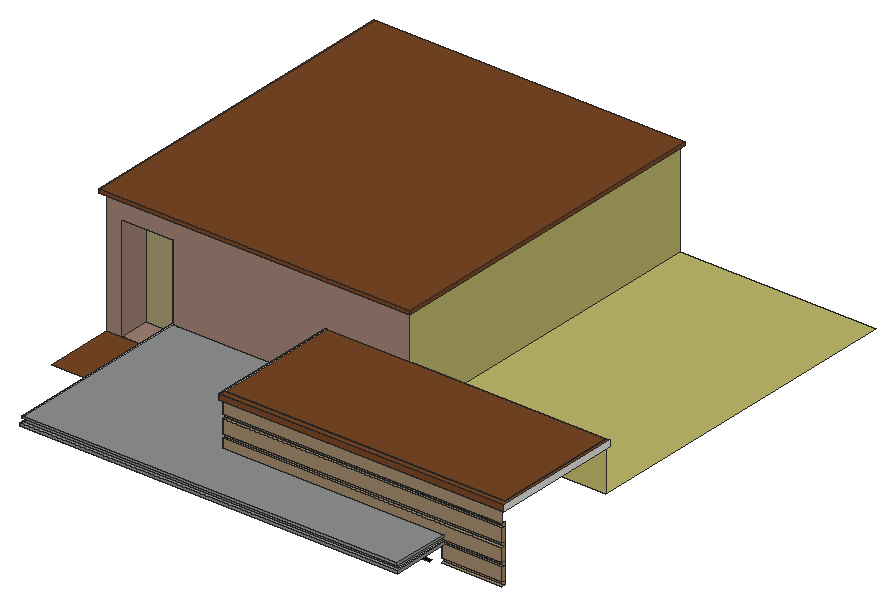
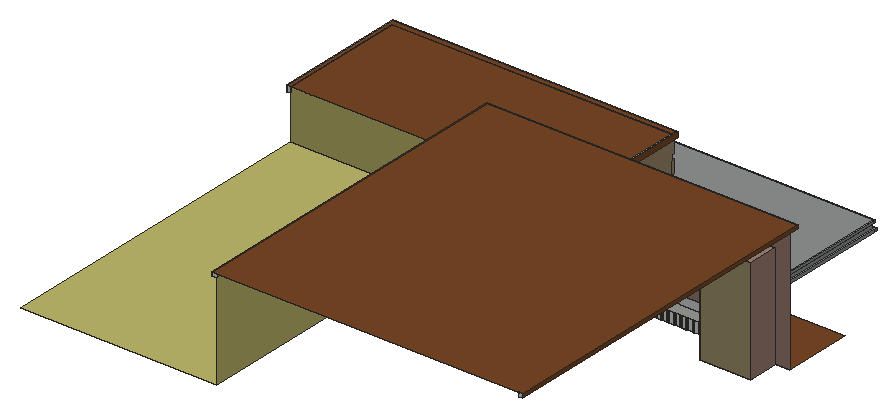
# SketchUp Ruby script. Lengths in inches.
U = 1.inch
M = Sketchup.active_model
def pt(a) = Geom::Point3d.new(a.map { |v| v * U })
def face(e, loops, mat)
  f = e.add_face(loops[0].map { |a| pt(a) })
  loops[1..].each { |l| e.add_face(l.map { |a| pt(a) }).erase! }
  f.material = f.back_material = mat if mat
  f
end
# faces: each face lists its corners as indices into pts; further lists are holes
def faces(e, pts, list, mat = nil) = list.each { |f| face(e, (f[0].is_a?(Array) ? f : [f]).map { |l| l.map { |i| pts[i] } }, mat) }
# xy, xz, yz: faces in a plane at the given z, y or x. An outline is a flat list of corners, or four numbers for a rectangle; further outlines are holes
def ring(l) = l.size == 4 ? [[l[0], l[1]], [l[2], l[1]], [l[2], l[3]], [l[0], l[3]]] : l.each_slice(2).to_a
def flat(e, list, mat, &to3) = list.each { |f| face(e, (f[0].is_a?(Array) ? f : [f]).map { |l| ring(l).map { |u, v| to3.(u, v) } }, mat) }
def xy(e, z, list, mat = nil) = flat(e, list, mat) { |x, y| [x, y, z] }
def xz(e, y, list, mat = nil) = flat(e, list, mat) { |x, z| [x, y, z] }
def yz(e, x, list, mat = nil) = flat(e, list, mat) { |y, z| [x, y, z] }
def lines(e, pts, list) = list.each { |a, b| e.add_line(pt(pts[a]), pt(pts[b])) }
# prism: a flat outline (further loops are holes) pulled along v
def prism(e, loops, v, mat = nil)
  f = face(e, loops, mat); d = Geom::Vector3d.new(v.map { |x| x * U })
  f.pushpull(f.normal.samedirection?(d) ? d.length : -d.length)
end
def box(e, o, s, mat = nil) = prism(e, [[o, [o[0] + s[0], o[1], o[2]], [o[0] + s[0], o[1] + s[1], o[2]], [o[0], o[1] + s[1], o[2]]]], [0, 0, s[2]], mat)
def at(x, y, z, deg = 0) = Geom::Transformation.translation(pt([x, y, z])) * Geom::Transformation.rotation(ORIGIN, Z_AXIS, deg.degrees)
def axes(o, x, y, z) = Geom::Transformation.new([*x, 0, *y, 0, *z, 0, *pt(o).to_a, 1])
def part(name) = M.definitions.add(name)
# library, detail: a bought-in or finely detailed component or shape, given as its bounding box
def library(name, o, s) = part(name).tap { |d| box(d.entities, o, s) }
def detail(e, o, s) = box(e.add_group.entities, o, s)
def put(e, d, t, mat = nil) = e.add_instance(d, t).tap { |i| i.material = mat if mat }
def group(e, t, mat = nil) = e.add_group.tap { |g| g.transformation = t; g.material = mat if mat }.entities
root = M.entities
M.materials.add("Niraj_Hair_Dark").color = [109, 109, 109]
M.materials.add("Niraj_Skin").color = [158, 128, 115]
M.materials.add("[0026_LightSalmon]").color = [255, 160, 122]
M.materials.add("[0035_Tan]").color = [158, 135, 105]
M.materials.add("[0057_DarkKhaki]").color = [189, 183, 107]
M.materials.add("[0137_Black]").color = [0, 0, 0]
M.materials.add("[Blacktop Old 02]").color = [143, 145, 145]
M.materials.add("[Wood Lumber ButtJoined]").color = [164, 152, 112]
M.materials.add("[Wood Veneer 01]").color = [120, 70, 37]
xy(root,249,[[18.5,262.5,71.22,294.13]],"Niraj_Skin")
xy(root,249.09,[[71.42,259.5,75.97,262.5],[77.92,259.5,82.47,262.5],[84.42,259.5,88.97,262.5],[90.92,259.5,95.47,262.5],[97.42,259.5,101.97,262.5],
  [103.92,259.5,108.47,262.5],[110.42,259.5,114.97,262.5],[116.92,259.5,121.47,262.5],[123.42,259.5,127.97,262.5],[129.92,259.5,134.47,262.5],
  [136.42,259.5,140.97,262.5],[142.92,259.5,147.47,262.5],[149.42,259.5,153.97,262.5],[155.92,259.5,160.47,262.5],[162.42,259.5,166.97,262.5],
  [168.92,259.5,173.47,262.5],[175.17,259.5,179.72,262.5],[181.42,259.5,185.97,262.5],[187.67,259.5,192.22,262.5],[193.92,259.5,198.47,262.5],
  [200.17,259.5,204.72,262.5],[206.42,259.5,210.97,262.5],[212.67,259.5,217.22,262.5],[218.92,259.5,223.47,262.5],[225.17,259.5,229.72,262.5],
  [231.42,259.5,235.97,262.5],[237.67,259.5,242.22,262.5],[243.92,259.5,248.47,262.5],[250.17,259.5,254.72,262.5],[256.42,259.5,260.97,262.5],
  [262.67,259.5,267.22,262.5],[269.11,259.5,273.65,262.5],[275.54,259.5,280.09,262.5],[281.98,259.5,286.53,262.5],[288.42,259.5,292.97,262.5],
  [294.86,259.5,299.4,262.5],[301.29,259.5,305.84,262.5]])
xy(root,249.09,[[3.5,191.32,310.1875,191.32,310.1875,262.5,305.84,262.5,305.84,259.5,301.29,259.5,301.29,262.5,299.4,262.5,299.4,259.5,294.86,259.5,294.86,262.5,292.97,262.5,292.97,259.5,288.42,259.5,288.42,262.5,286.53,262.5,286.53,259.5,281.98,259.5,281.98,262.5,280.09,262.5,280.09,259.5,275.54,259.5,275.54,262.5,273.65,262.5,273.65,259.5,269.11,259.5,269.11,262.5,267.22,262.5,267.22,259.5,262.67,259.5,262.67,262.5,260.97,262.5,260.97,259.5,256.42,259.5,256.42,262.5,254.72,262.5,254.72,259.5,250.17,259.5,250.17,262.5,248.47,262.5,248.47,259.5,243.92,259.5,243.92,262.5,242.22,262.5,242.22,259.5,237.67,259.5,237.67,262.5,235.97,262.5,235.97,259.5,231.42,259.5,231.42,262.5,229.72,262.5,229.72,259.5,225.17,259.5,225.17,262.5,223.47,262.5,223.47,259.5,218.92,259.5,218.92,262.5,217.22,262.5,217.22,259.5,212.67,259.5,212.67,262.5,210.97,262.5,210.97,259.5,206.42,259.5,206.42,262.5,204.72,262.5,204.72,259.5,200.17,259.5,200.17,262.5,198.47,262.5,198.47,259.5,193.92,259.5,193.92,262.5,192.22,262.5,192.22,259.5,187.67,259.5,187.67,262.5,185.97,262.5,185.97,259.5,181.42,259.5,181.42,262.5,179.72,262.5,179.72,259.5,175.17,259.5,175.17,262.5,173.47,262.5,173.47,259.5,168.92,259.5,168.92,262.5,166.97,262.5,166.97,259.5,162.42,259.5,162.42,262.5,160.47,262.5,160.47,259.5,155.92,259.5,155.92,262.5,153.97,262.5,153.97,259.5,149.42,259.5,149.42,262.5,147.47,262.5,147.47,259.5,142.92,259.5,142.92,262.5,140.97,262.5,140.97,259.5,136.42,259.5,136.42,262.5,134.47,262.5,134.47,259.5,129.92,259.5,129.92,262.5,127.97,262.5,127.97,259.5,123.42,259.5,123.42,262.5,121.47,262.5,121.47,259.5,116.92,259.5,116.92,262.5,114.97,262.5,114.97,259.5,110.42,259.5,110.42,262.5,108.47,262.5,108.47,259.5,103.92,259.5,103.92,262.5,101.97,262.5,101.97,259.5,97.42,259.5,97.42,262.5,95.47,262.5,95.47,259.5,90.92,259.5,90.92,262.5,88.97,262.5,88.97,259.5,84.42,259.5,84.42,262.5,82.47,262.5,82.47,259.5,77.92,259.5,77.92,262.5,75.97,262.5,75.97,259.5,71.42,259.5,71.42,262.5,3.5,262.5]],"[Wood Veneer 01]")
xy(root,249.27,[[367.23,128.5,444.17,131.5]],"[0137_Black]")
xy(root,252.4375,[[456.23,128.5,518.75,131.5]],"[0035_Tan]")
xy(root,256.58,[[456.23,128.5,518.75,131.5]],"[0035_Tan]")
xy(root,269.38,[[71.42,259.5,75.97,262.5],[77.92,259.5,82.47,262.5],[84.42,259.5,88.97,262.5],[90.92,259.5,95.47,262.5],[97.42,259.5,101.97,262.5],
  [103.92,259.5,108.47,262.5],[110.42,259.5,114.97,262.5],[116.92,259.5,121.47,262.5],[123.42,259.5,127.97,262.5],[129.92,259.5,134.47,262.5],
  [136.42,259.5,140.97,262.5],[142.92,259.5,147.47,262.5],[149.42,259.5,153.97,262.5],[155.92,259.5,160.47,262.5],[162.42,259.5,166.97,262.5],
  [168.92,259.5,173.47,262.5],[175.17,259.5,179.72,262.5],[181.42,259.5,185.97,262.5],[187.67,259.5,192.22,262.5],[193.92,259.5,198.47,262.5],
  [200.17,259.5,204.72,262.5],[206.42,259.5,210.97,262.5],[212.67,259.5,217.22,262.5],[218.92,259.5,223.47,262.5],[225.17,259.5,229.72,262.5],
  [231.42,259.5,235.97,262.5],[237.67,259.5,242.22,262.5],[243.92,259.5,248.47,262.5],[250.17,259.5,254.72,262.5],[256.42,259.5,260.97,262.5],
  [262.67,259.5,267.22,262.5],[269.11,259.5,273.65,262.5],[275.54,259.5,280.09,262.5],[281.98,259.5,286.53,262.5],[288.42,259.5,292.97,262.5],
  [294.86,259.5,299.4,262.5],[301.29,259.5,305.84,262.5]])
xy(root,269.38,[[69.11,68.5,69.11,262.5,71.42,262.5,71.42,259.5,75.97,259.5,75.97,262.5,77.04,262.5,77.04,274.5,310.1875,274.5,310.1875,131.5,445.29,131.5,445.29,71.5,456.23,71.5,456.23,128.5,458.66,128.5,458.66,68.5]],"[Blacktop Old 02]")
xy(root,270.4375,[[456.23,128.5,518.75,131.5]],"[0035_Tan]")
xy(root,272.21,[[69.11,68.5,458.66,68.5,458.66,128.5,456.23,128.5,456.23,71.5,71.42,71.5,71.42,262.5,69.11,262.5]],"[Blacktop Old 02]")
xy(root,274.58,[[456.23,128.5,518.75,131.5]],"[0035_Tan]")
xy(root,276.6875,[[70.17,68.5,70.17,262.5,71.42,262.5,71.42,71.5,456.23,71.5,456.23,128.5,457.98,128.5,457.98,68.5]],"Niraj_Hair_Dark")
xy(root,279,[[230.1,128.5,456.23,131.5]])
xy(root,279,[[70.17,68.5,71.42,71.5]],"Niraj_Hair_Dark")
xy(root,279,[[316.1875,262.5,518.75,611.5]],"[0057_DarkKhaki]")
xy(root,279,[[71.42,68.5,457.98,68.5,457.98,128.5,230.1,128.5,230.1,262.5,310.1875,262.5,310.1875,274.5,77.04,274.5,77.04,262.5,71.42,262.5],[70.17,71.5,71.42,262.5]],"[Blacktop Old 02]")
xy(root,288.4375,[[230.1,128.5,518.75,131.5]],"[0035_Tan]")
xy(root,292.58,[[230.1,128.5,518.75,131.5]],"[0035_Tan]")
xy(root,306.4375,[[230.1,128.5,518.75,131.5]],"[0035_Tan]")
xy(root,310.58,[[230.1,128.5,518.75,131.5]],"[0035_Tan]")
xy(root,324.4375,[[230.1,128.5,518.75,131.5]])
xy(root,324.4375,[[228.35,125.5,228.35,262.5,230.1,262.5,230.1,128.5,518.75,128.5,518.75,262.5,522.9375,262.5,522.9375,125.5]],"[Wood Veneer 01]")
xy(root,330.3125,[[228.35,125.5,230.1,131.5],[230.1,125.5,522.9375,125.5,522.9375,262.5,518.75,262.5,518.75,131.5,230.1,131.5],[228.35,131.5,230.1,262.5],[230.1,131.5,518.75,262.5]],"[Wood Veneer 01]")
xy(root,357,[[18.5,262.5,71.22,294.13]],"Niraj_Skin")
xy(root,377.89,[[0,256.5,0,611.5,3.5,611.5,3.5,262.5,316.1875,262.5,316.1875,611.5,320.5,611.5,320.5,256.5]],"[Wood Veneer 01]")
xy(root,381.875,[[0,256.5,320.5,611.5]],"[Wood Veneer 01]")
xz(root,68.5,[[69.11,269.38,458.66,272.21],[70.17,276.6875,457.98,279]],"[Blacktop Old 02]")
xz(root,71.5,[[71.42,272.21,456.23,276.6875]],"[Blacktop Old 02]")
xz(root,125.5,[[228.35,324.4375,522.9375,330.3125]],"[Wood Veneer 01]")
xz(root,128.5,[[456.23,269.38,458.66,270.4375],[456.23,270.4375,458.66,272.21]])
xz(root,128.5,[[456.23,256.58,518.75,256.58,518.75,270.4375,458.66,270.4375,458.66,269.38,456.23,269.38],[456.23,274.58,518.75,274.58,518.75,288.4375,230.1,288.4375,230.1,279,457.98,279,457.98,276.6875,456.23,276.6875],[230.1,292.58,518.75,306.4375],[230.1,310.58,518.75,324.4375]],"[0035_Tan]")
xz(root,131.5,[[456.23,256.58,518.75,270.4375],[230.1,274.58,456.23,279],[456.23,274.58,456.23,279,230.1,279,230.1,288.4375,518.75,288.4375,518.75,274.58],[230.1,292.58,518.75,306.4375],[230.1,324.4375,518.75,330.3125]])
xz(root,131.5,[[456.23,252.4375,518.75,256.58],[456.23,270.4375,518.75,274.58],[230.1,288.4375,518.75,292.58],[230.1,306.4375,518.75,310.58]],"[0035_Tan]")
xz(root,256.5,[[0,377.89,320.5,381.875]],"[Wood Veneer 01]")
xz(root,259.5,[[71.42,249.09,75.97,269.38],[77.92,249.09,82.47,269.38],[84.42,249.09,88.97,269.38],[90.92,249.09,95.47,269.38],[97.42,249.09,101.97,269.38],
  [103.92,249.09,108.47,269.38],[110.42,249.09,114.97,269.38],[116.92,249.09,121.47,269.38],[123.42,249.09,127.97,269.38],[129.92,249.09,134.47,269.38],
  [136.42,249.09,140.97,269.38],[142.92,249.09,147.47,269.38],[149.42,249.09,153.97,269.38],[155.92,249.09,160.47,269.38],[162.42,249.09,166.97,269.38],
  [168.92,249.09,173.47,269.38],[175.17,249.09,179.72,269.38],[181.42,249.09,185.97,269.38],[187.67,249.09,192.22,269.38],[193.92,249.09,198.47,269.38],
  [200.17,249.09,204.72,269.38],[206.42,249.09,210.97,269.38],[212.67,249.09,217.22,269.38],[218.92,249.09,223.47,269.38],[225.17,249.09,229.72,269.38],
  [231.42,249.09,235.97,269.38],[237.67,249.09,242.22,269.38],[243.92,249.09,248.47,269.38],[250.17,249.09,254.72,269.38],[256.42,249.09,260.97,269.38],
  [262.67,249.09,267.22,269.38],[269.11,249.09,273.65,269.38],[275.54,249.09,280.09,269.38],[281.98,249.09,286.53,269.38],[288.42,249.09,292.97,269.38],
  [294.86,249.09,299.4,269.38],[301.29,249.09,305.84,269.38]],"[0026_LightSalmon]")
xz(root,262.5,[[18.5,249,71.22,249.09],[71.42,249.09,75.97,269.38],[77.92,249.09,82.47,269.38],[84.42,249.09,88.97,269.38],[90.92,249.09,95.47,269.38],
  [97.42,249.09,101.97,269.38],[103.92,249.09,108.47,269.38],[110.42,249.09,114.97,269.38],[116.92,249.09,121.47,269.38],[123.42,249.09,127.97,269.38],
  [129.92,249.09,134.47,269.38],[136.42,249.09,140.97,269.38],[142.92,249.09,147.47,269.38],[149.42,249.09,153.97,269.38],[155.92,249.09,160.47,269.38],
  [162.42,249.09,166.97,269.38],[168.92,249.09,173.47,269.38],[175.17,249.09,179.72,269.38],[181.42,249.09,185.97,269.38],[187.67,249.09,192.22,269.38],
  [193.92,249.09,198.47,269.38],[200.17,249.09,204.72,269.38],[206.42,249.09,210.97,269.38],[212.67,249.09,217.22,269.38],[218.92,249.09,223.47,269.38],
  [225.17,249.09,229.72,269.38],[231.42,249.09,235.97,269.38],[237.67,249.09,242.22,269.38],[243.92,249.09,248.47,269.38],[250.17,249.09,254.72,269.38],
  [256.42,249.09,260.97,269.38],[262.67,249.09,267.22,269.38],[269.11,249.09,273.65,269.38],[275.54,249.09,280.09,269.38],[281.98,249.09,286.53,269.38],
  [288.42,249.09,292.97,269.38],[294.86,249.09,299.4,269.38],[301.29,249.09,305.84,269.38],[69.11,269.38,71.22,272.21],[71.22,269.38,71.42,272.21],
  [71.42,269.38,77.04,279],[71.22,272.21,71.42,276.6875],[70.17,276.6875,71.22,279],[71.22,276.6875,71.42,279],[230.1,279,310.1875,330.3125],
  [518.75,324.4375,522.9375,330.3125]])
xz(root,262.5,[[3.5,249.09,18.5,249.09,18.5,357,71.22,357,71.22,279,77.04,279,77.04,269.38,75.97,269.38,75.97,249.09,77.92,249.09,77.92,269.38,82.47,269.38,82.47,249.09,84.42,249.09,84.42,269.38,88.97,269.38,88.97,249.09,90.92,249.09,90.92,269.38,95.47,269.38,95.47,249.09,97.42,249.09,97.42,269.38,101.97,269.38,101.97,249.09,103.92,249.09,103.92,269.38,108.47,269.38,108.47,249.09,110.42,249.09,110.42,269.38,114.97,269.38,114.97,249.09,116.92,249.09,116.92,269.38,121.47,269.38,121.47,249.09,123.42,249.09,123.42,269.38,127.97,269.38,127.97,249.09,129.92,249.09,129.92,269.38,134.47,269.38,134.47,249.09,136.42,249.09,136.42,269.38,140.97,269.38,140.97,249.09,142.92,249.09,142.92,269.38,147.47,269.38,147.47,249.09,149.42,249.09,149.42,269.38,153.97,269.38,153.97,249.09,155.92,249.09,155.92,269.38,160.47,269.38,160.47,249.09,162.42,249.09,162.42,269.38,166.97,269.38,166.97,249.09,168.92,249.09,168.92,269.38,173.47,269.38,173.47,249.09,175.17,249.09,175.17,269.38,179.72,269.38,179.72,249.09,181.42,249.09,181.42,269.38,185.97,269.38,185.97,249.09,187.67,249.09,187.67,269.38,192.22,269.38,192.22,249.09,193.92,249.09,193.92,269.38,198.47,269.38,198.47,249.09,200.17,249.09,200.17,269.38,204.72,269.38,204.72,249.09,206.42,249.09,206.42,269.38,210.97,269.38,210.97,249.09,212.67,249.09,212.67,269.38,217.22,269.38,217.22,249.09,218.92,249.09,218.92,269.38,223.47,269.38,223.47,249.09,225.17,249.09,225.17,269.38,229.72,269.38,229.72,249.09,231.42,249.09,231.42,269.38,235.97,269.38,235.97,249.09,237.67,249.09,237.67,269.38,242.22,269.38,242.22,249.09,243.92,249.09,243.92,269.38,248.47,269.38,248.47,249.09,250.17,249.09,250.17,269.38,254.72,269.38,254.72,249.09,256.42,249.09,256.42,269.38,260.97,269.38,260.97,249.09,262.67,249.09,262.67,269.38,267.22,269.38,267.22,249.09,269.11,249.09,269.11,269.38,273.65,269.38,273.65,249.09,275.54,249.09,275.54,269.38,280.09,269.38,280.09,249.09,281.98,249.09,281.98,269.38,286.53,269.38,286.53,249.09,288.42,249.09,288.42,269.38,292.97,269.38,292.97,249.09,294.86,249.09,294.86,269.38,299.4,269.38,299.4,249.09,301.29,249.09,301.29,269.38,305.84,269.38,305.84,249.09,310.1875,249.09,310.1875,279,230.1,279,230.1,324.4375,228.35,324.4375,228.35,330.3125,316.1875,330.3125,316.1875,377.89,3.5,377.89]],"Niraj_Skin")
xz(root,262.5,[[71.22,249.09,71.42,269.38]],"[0026_LightSalmon]")
xz(root,262.5,[[316.1875,279,518.75,330.3125]],"[0057_DarkKhaki]")
xz(root,274.5,[[77.04,269.38,310.1875,279]])
xz(root,294.13,[[18.5,249,71.22,357]],"[Wood Lumber ButtJoined]")
xz(root,611.5,[[0,377.89,3.5,381.875],[316.1875,377.89,320.5,381.875]])
yz(root,0,[[256.5,377.89,611.5,381.875]],"[Wood Veneer 01]")
yz(root,18.5,[[262.5,249,294.13,357]],"Niraj_Skin")
yz(root,69.11,[[68.5,269.38,71.5,272.21]],"Niraj_Hair_Dark")
yz(root,69.11,[[71.5,269.38,262.5,272.21]],"[Blacktop Old 02]")
yz(root,70.17,[[68.5,276.6875,71.5,279]],"Niraj_Hair_Dark")
yz(root,70.17,[[71.5,276.6875,262.5,279]],"[Blacktop Old 02]")
yz(root,71.22,[[262.5,249,294.13,357]],"Niraj_Skin")
yz(root,71.42,[[71.5,276.6875,262.5,279]])
yz(root,71.42,[[259.5,249.09,262.5,269.38]],"[0026_LightSalmon]")
yz(root,71.42,[[71.5,272.21,262.5,276.6875]],"[Blacktop Old 02]")
yz(root,75.97,[[259.5,249.09,262.5,269.38]],"[0026_LightSalmon]")
yz(root,77.04,[[262.5,269.38,274.5,279]])
yz(root,77.92,[[259.5,249.09,262.5,269.38]],"[0026_LightSalmon]")
yz(root,82.47,[[259.5,249.09,262.5,269.38]],"[0026_LightSalmon]")
yz(root,84.42,[[259.5,249.09,262.5,269.38]],"[0026_LightSalmon]")
yz(root,88.97,[[259.5,249.09,262.5,269.38]],"[0026_LightSalmon]")
yz(root,90.92,[[259.5,249.09,262.5,269.38]],"[0026_LightSalmon]")
yz(root,95.47,[[259.5,249.09,262.5,269.38]],"[0026_LightSalmon]")
yz(root,97.42,[[259.5,249.09,262.5,269.38]],"[0026_LightSalmon]")
yz(root,101.97,[[259.5,249.09,262.5,269.38]],"[0026_LightSalmon]")
yz(root,103.92,[[259.5,249.09,262.5,269.38]],"[0026_LightSalmon]")
yz(root,108.47,[[259.5,249.09,262.5,269.38]],"[0026_LightSalmon]")
yz(root,110.42,[[259.5,249.09,262.5,269.38]],"[0026_LightSalmon]")
yz(root,114.97,[[259.5,249.09,262.5,269.38]],"[0026_LightSalmon]")
yz(root,116.92,[[259.5,249.09,262.5,269.38]],"[0026_LightSalmon]")
yz(root,121.47,[[259.5,249.09,262.5,269.38]],"[0026_LightSalmon]")
yz(root,123.42,[[259.5,249.09,262.5,269.38]],"[0026_LightSalmon]")
yz(root,127.97,[[259.5,249.09,262.5,269.38]],"[0026_LightSalmon]")
yz(root,129.92,[[259.5,249.09,262.5,269.38]],"[0026_LightSalmon]")
yz(root,134.47,[[259.5,249.09,262.5,269.38]],"[0026_LightSalmon]")
yz(root,136.42,[[259.5,249.09,262.5,269.38]],"[0026_LightSalmon]")
yz(root,140.97,[[259.5,249.09,262.5,269.38]],"[0026_LightSalmon]")
yz(root,142.92,[[259.5,249.09,262.5,269.38]],"[0026_LightSalmon]")
yz(root,147.47,[[259.5,249.09,262.5,269.38]],"[0026_LightSalmon]")
yz(root,149.42,[[259.5,249.09,262.5,269.38]],"[0026_LightSalmon]")
yz(root,153.97,[[259.5,249.09,262.5,269.38]],"[0026_LightSalmon]")
yz(root,155.92,[[259.5,249.09,262.5,269.38]],"[0026_LightSalmon]")
yz(root,160.47,[[259.5,249.09,262.5,269.38]],"[0026_LightSalmon]")
yz(root,162.42,[[259.5,249.09,262.5,269.38]],"[0026_LightSalmon]")
yz(root,166.97,[[259.5,249.09,262.5,269.38]],"[0026_LightSalmon]")
yz(root,168.92,[[259.5,249.09,262.5,269.38]],"[0026_LightSalmon]")
yz(root,173.47,[[259.5,249.09,262.5,269.38]],"[0026_LightSalmon]")
yz(root,175.17,[[259.5,249.09,262.5,269.38]],"[0026_LightSalmon]")
yz(root,179.72,[[259.5,249.09,262.5,269.38]],"[0026_LightSalmon]")
yz(root,181.42,[[259.5,249.09,262.5,269.38]],"[0026_LightSalmon]")
yz(root,185.97,[[259.5,249.09,262.5,269.38]],"[0026_LightSalmon]")
yz(root,187.67,[[259.5,249.09,262.5,269.38]],"[0026_LightSalmon]")
yz(root,192.22,[[259.5,249.09,262.5,269.38]],"[0026_LightSalmon]")
yz(root,193.92,[[259.5,249.09,262.5,269.38]],"[0026_LightSalmon]")
yz(root,198.47,[[259.5,249.09,262.5,269.38]],"[0026_LightSalmon]")
yz(root,200.17,[[259.5,249.09,262.5,269.38]],"[0026_LightSalmon]")
yz(root,204.72,[[259.5,249.09,262.5,269.38]],"[0026_LightSalmon]")
yz(root,206.42,[[259.5,249.09,262.5,269.38]],"[0026_LightSalmon]")
yz(root,210.97,[[259.5,249.09,262.5,269.38]],"[0026_LightSalmon]")
yz(root,212.67,[[259.5,249.09,262.5,269.38]],"[0026_LightSalmon]")
yz(root,217.22,[[259.5,249.09,262.5,269.38]],"[0026_LightSalmon]")
yz(root,218.92,[[259.5,249.09,262.5,269.38]],"[0026_LightSalmon]")
yz(root,223.47,[[259.5,249.09,262.5,269.38]],"[0026_LightSalmon]")
yz(root,225.17,[[259.5,249.09,262.5,269.38]],"[0026_LightSalmon]")
yz(root,228.35,[[125.5,324.4375,262.5,330.3125]],"[Wood Veneer 01]")
yz(root,229.72,[[259.5,249.09,262.5,269.38]],"[0026_LightSalmon]")
yz(root,230.1,[[131.5,324.4375,262.5,330.3125]])
yz(root,230.1,[[128.5,279,131.5,288.4375],[131.5,279,131.5,310.58,128.5,310.58,128.5,324.4375,262.5,324.4375,262.5,279],[128.5,292.58,131.5,306.4375]],"[0035_Tan]")
yz(root,231.42,[[259.5,249.09,262.5,269.38]],"[0026_LightSalmon]")
yz(root,235.97,[[259.5,249.09,262.5,269.38]],"[0026_LightSalmon]")
yz(root,237.67,[[259.5,249.09,262.5,269.38]],"[0026_LightSalmon]")
yz(root,242.22,[[259.5,249.09,262.5,269.38]],"[0026_LightSalmon]")
yz(root,243.92,[[259.5,249.09,262.5,269.38]],"[0026_LightSalmon]")
yz(root,248.47,[[259.5,249.09,262.5,269.38]],"[0026_LightSalmon]")
yz(root,250.17,[[259.5,249.09,262.5,269.38]],"[0026_LightSalmon]")
yz(root,254.72,[[259.5,249.09,262.5,269.38]],"[0026_LightSalmon]")
yz(root,256.42,[[259.5,249.09,262.5,269.38]],"[0026_LightSalmon]")
yz(root,260.97,[[259.5,249.09,262.5,269.38]],"[0026_LightSalmon]")
yz(root,262.67,[[259.5,249.09,262.5,269.38]],"[0026_LightSalmon]")
yz(root,267.22,[[259.5,249.09,262.5,269.38]],"[0026_LightSalmon]")
yz(root,269.11,[[259.5,249.09,262.5,269.38]],"[0026_LightSalmon]")
yz(root,273.65,[[259.5,249.09,262.5,269.38]],"[0026_LightSalmon]")
yz(root,275.54,[[259.5,249.09,262.5,269.38]],"[0026_LightSalmon]")
yz(root,280.09,[[259.5,249.09,262.5,269.38]],"[0026_LightSalmon]")
yz(root,281.98,[[259.5,249.09,262.5,269.38]],"[0026_LightSalmon]")
yz(root,286.53,[[259.5,249.09,262.5,269.38]],"[0026_LightSalmon]")
yz(root,288.42,[[259.5,249.09,262.5,269.38]],"[0026_LightSalmon]")
yz(root,292.97,[[259.5,249.09,262.5,269.38]],"[0026_LightSalmon]")
yz(root,294.86,[[259.5,249.09,262.5,269.38]],"[0026_LightSalmon]")
yz(root,299.4,[[259.5,249.09,262.5,269.38]],"[0026_LightSalmon]")
yz(root,301.29,[[259.5,249.09,262.5,269.38]],"[0026_LightSalmon]")
yz(root,305.84,[[259.5,249.09,262.5,269.38]])
yz(root,310.1875,[[262.5,269.38,268.5,279],[268.5,269.38,274.5,279]])
yz(root,316.1875,[[262.5,279,611.5,377.89]],"[0057_DarkKhaki]")
yz(root,320.5,[[256.5,377.89,611.5,381.875]],"[Wood Veneer 01]")
yz(root,456.23,[[128.5,256.58,131.5,270.4375],[71.5,269.38,128.5,272.21],[128.5,274.58,131.5,279]])
yz(root,456.23,[[128.5,270.4375,131.5,270.4375,131.5,274.58,128.5,274.58,128.5,276.6875,71.5,276.6875,71.5,272.21,128.5,272.21]],"[Blacktop Old 02]")
yz(root,457.98,[[68.5,276.6875,128.5,279]],"[Blacktop Old 02]")
yz(root,458.66,[[68.5,269.38,128.5,272.21]],"[Blacktop Old 02]")
yz(root,518.75,[[131.5,324.4375,262.5,330.3125]])
yz(root,518.75,[[128.5,256.58,131.5,270.4375],[128.5,274.58,131.5,288.4375],[128.5,292.58,131.5,306.4375]],"[0035_Tan]")
yz(root,522.9375,[[125.5,324.4375,262.5,330.3125]])
p = [[310.1875,268.5,279],[310.1875,268.5,363],[77.04,262.5,269.38],[77.04,262.5,269.25],[71.42,71.5,269.38],[71.42,71.5,272.21],
  [456.23,131.5,256.58],[445.29,131.5,256.58],[3.5,262.5,377.89],[3.5,262.5,381.875],[316.1875,268.5,377.89],[316.1875,268.5,381.875]]
lines(root,p,[[0,1],[2,3],[4,5],[6,7],[8,9],[10,11]])
